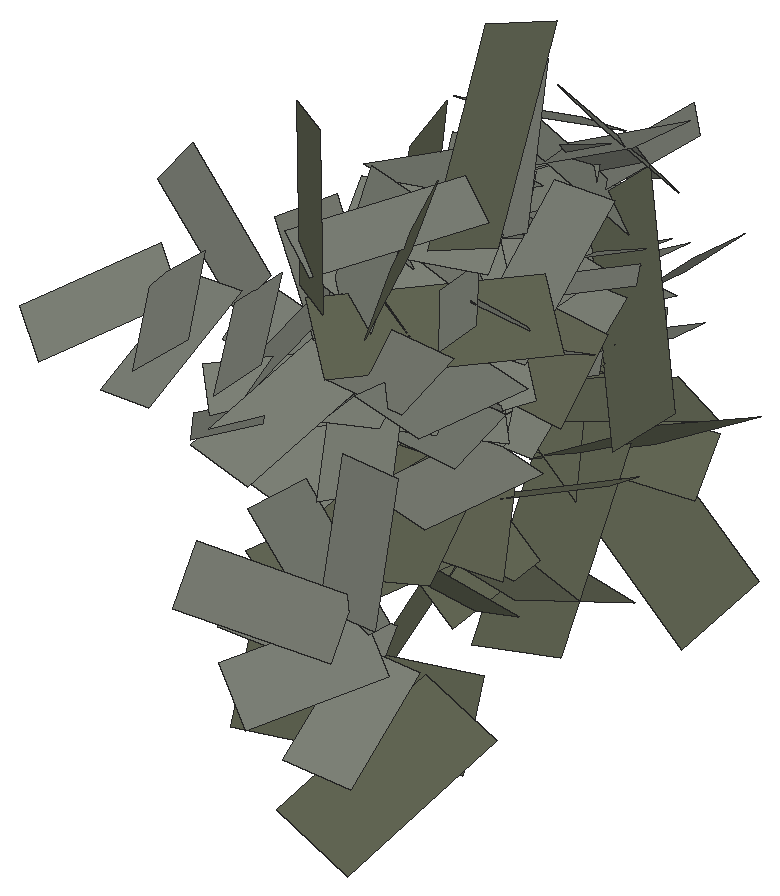
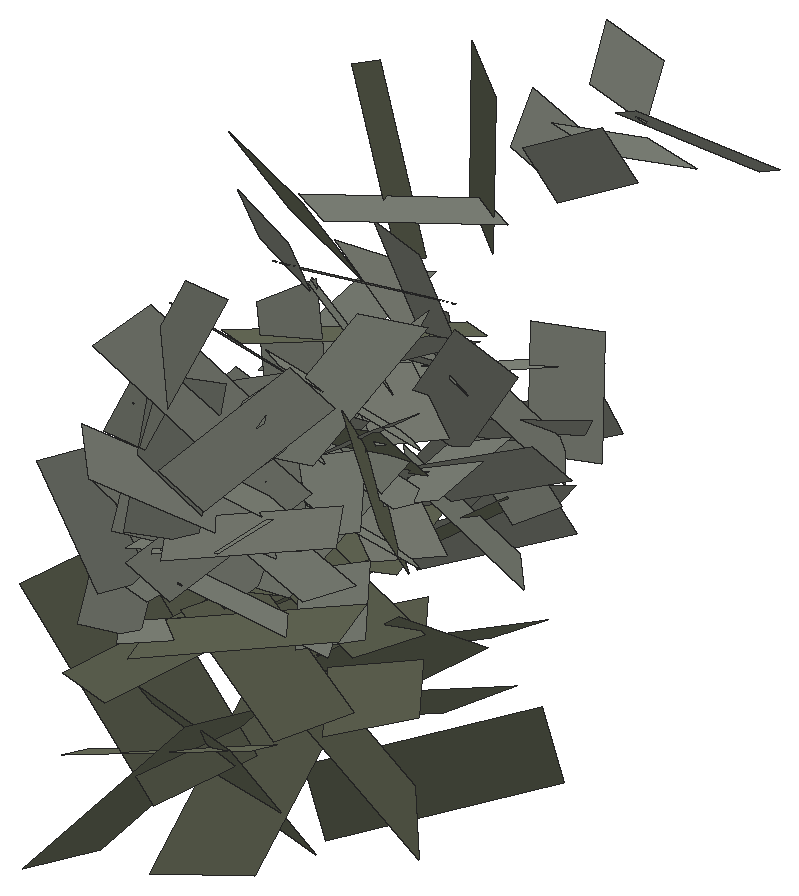
# SketchUp Ruby script. Lengths in inches.
U = 1.inch
M = Sketchup.active_model
def pt(a) = Geom::Point3d.new(a.map { |v| v * U })
def face(e, loops, mat)
  f = e.add_face(loops[0].map { |a| pt(a) })
  loops[1..].each { |l| e.add_face(l.map { |a| pt(a) }).erase! }
  f.material = f.back_material = mat if mat
  f
end
# faces: each face lists its corners as indices into pts; further lists are holes
def faces(e, pts, list, mat = nil) = list.each { |f| face(e, (f[0].is_a?(Array) ? f : [f]).map { |l| l.map { |i| pts[i] } }, mat) }
# xy, xz, yz: faces in a plane at the given z, y or x. An outline is a flat list of corners, or four numbers for a rectangle; further outlines are holes
def ring(l) = l.size == 4 ? [[l[0], l[1]], [l[2], l[1]], [l[2], l[3]], [l[0], l[3]]] : l.each_slice(2).to_a
def flat(e, list, mat, &to3) = list.each { |f| face(e, (f[0].is_a?(Array) ? f : [f]).map { |l| ring(l).map { |u, v| to3.(u, v) } }, mat) }
def xy(e, z, list, mat = nil) = flat(e, list, mat) { |x, y| [x, y, z] }
def xz(e, y, list, mat = nil) = flat(e, list, mat) { |x, z| [x, y, z] }
def yz(e, x, list, mat = nil) = flat(e, list, mat) { |y, z| [x, y, z] }
def lines(e, pts, list) = list.each { |a, b| e.add_line(pt(pts[a]), pt(pts[b])) }
# prism: a flat outline (further loops are holes) pulled along v
def prism(e, loops, v, mat = nil)
  f = face(e, loops, mat); d = Geom::Vector3d.new(v.map { |x| x * U })
  f.pushpull(f.normal.samedirection?(d) ? d.length : -d.length)
end
def box(e, o, s, mat = nil) = prism(e, [[o, [o[0] + s[0], o[1], o[2]], [o[0] + s[0], o[1] + s[1], o[2]], [o[0], o[1] + s[1], o[2]]]], [0, 0, s[2]], mat)
def at(x, y, z, deg = 0) = Geom::Transformation.translation(pt([x, y, z])) * Geom::Transformation.rotation(ORIGIN, Z_AXIS, deg.degrees)
def axes(o, x, y, z) = Geom::Transformation.new([*x, 0, *y, 0, *z, 0, *pt(o).to_a, 1])
def part(name) = M.definitions.add(name)
# library, detail: a bought-in or finely detailed component or shape, given as its bounding box
def library(name, o, s) = part(name).tap { |d| box(d.entities, o, s) }
def detail(e, o, s) = box(e.add_group.entities, o, s)
def put(e, d, t, mat = nil) = e.add_instance(d, t).tap { |i| i.material = mat if mat }
def group(e, t, mat = nil) = e.add_group.tap { |g| g.transformation = t; g.material = mat if mat }.entities
root = M.entities
M.materials.add("viburnumblaasdfas0df1w06d").color = [98, 102, 84]
M.materials.add("viburnumbladsadfasdfad0w122").color = [125, 129, 119]
c1 = part("Component\#315")
p = [[0.25,0,0],[2.05,0.01,0.35],[1.81,4.2,1.66],[0,4.19,1.3125]]
faces(c1.entities,p,[[0,1,2,3]],"viburnumbladsadfasdfad0w122")
c2 = part("viburnumblad2")
put(c2.entities,c1,axes([-19.23,-4.49,-32.18],[83.35428,0,0],[0,79.38502,0],[0,0,83.35428]))
c3 = part("Component\#314")
p = [[0.14,0,0],[2.58,0.05,0.25],[2.44,5.11,2.64],[0,5.05,2.39]]
faces(c3.entities,p,[[0,1,2,3]],"viburnumblaasdfas0df1w06d")
c4 = part("viburnumblad1\#2")
put(c4.entities,c3,axes([-37.25,6.23,19.31],[75.98784,0,0],[0,65.50676,0],[0,0,75.98784]))
put(root,c2,axes([2206.21,336.26,21.66],[0.00219,0.00955,0.00743],[-0.01307,0.00092,0.00265],[0.0015,-0.00837,0.01031]))
put(root,c4,axes([2205.43,338.76,20.89],[0.01183,-0.00442,0.01203],[-0.00182,0.01827,0.0085],[-0.01272,-0.00605,0.01028]))
put(root,c2,axes([2206.37,328.02,29.41],[-0.00814,0.00715,0.0046],[-0.00805,-0.00423,-0.00746],[-0.00268,-0.00803,0.00677]))
put(root,c2,axes([2204.18,344.4,21.67],[-0.01,-0.00652,-0.00001],[0.00542,-0.00831,-0.00274],[0.00166,-0.00256,0.01102]))
put(root,c2,axes([2202.71,334.87,22.83],[0.00888,-0.0091,-0.0009],[0.00823,0.00741,0.00631],[-0.00398,-0.00497,0.01104]))
put(root,c2,axes([2205.18,339.76,23.52],[-0.01211,-0.00173,0.00211],[0.00069,-0.01077,-0.00395],[0.00303,-0.00413,0.011]))
put(root,c2,axes([2206.93,346.05,25.19],[-0.0062,0.01038,-0.0034],[-0.01088,-0.00717,-0.00204],[-0.00346,0.00185,0.01194]))
put(root,c2,axes([2205.36,335.66,23.13],[0.01106,0.0052,0.00541],[-0.00756,0.007,0.00872],[0.00055,-0.01018,0.00865]))
put(root,c2,axes([2204.26,334.51,23.09],[-0.00865,-0.00796,-0.00491],[0.00846,-0.00952,0.00054],[-0.00401,-0.0029,0.01175]))
put(root,c2,axes([2202.83,344.76,22.0625],[0.00554,-0.00849,-0.00419],[0.01058,0.00621,0.0014],[0.00119,-0.0044,0.01049]))
put(root,c2,axes([2203.29,335.87,20],[0.00852,-0.00783,-0.00192],[0.00823,0.00741,0.00631],[-0.003,-0.00593,0.01088]))
put(root,c4,axes([2208.25,345.48,20.74],[-0.00473,0.01294,-0.00003],[-0.01473,-0.00539,-0.00308],[-0.0025,-0.00088,0.01352]))
put(root,c2,axes([2207.21,335.39,22.89],[-0.00749,0.00812,0.00752],[-0.01012,-0.00577,-0.00385],[0.00099,-0.00855,0.01022]))
put(root,c2,axes([2206.23,330.56,27.9],[0.00736,0.00309,0.0079],[-0.00921,0.00654,0.0057],[-0.00262,-0.00929,0.00521]))
put(root,c4,axes([2203.95,342.96,17.85],[-0.0111,-0.00766,0.00199],[0.00742,-0.01279,-0.00569],[0.00489,-0.00308,0.01206]))
put(root,c2,axes([2203.05,340.66,22.82],[0.00848,-0.00639,-0.00524],[0.0093,0.00903,0.00402],[0.00207,-0.0066,0.01002]))
put(root,c2,axes([2204.8125,343.71,24.35],[-0.00958,-0.00624,-0.00001],[0.00602,-0.00923,-0.00305],[0.00166,-0.00256,0.01102]))
put(root,c2,axes([2206.84,346.58,26.86],[-0.01136,0.00239,-0.0048],[-0.00314,-0.01208,0.00143],[-0.00434,0.00249,0.01152]))
put(root,c2,axes([2204.6,340.74,22.52],[-0.00866,-0.0095,-0.00259],[0.00823,-0.00655,-0.00374],[0.002,-0.00468,0.01099]))
put(root,c2,axes([2206.52,343.58,26.43],[-0.01523,0.00004,-0.00037],[-0.00005,-0.01523,0.00032],[-0.00037,0.00032,0.01523]))
put(root,c4,axes([2203.32,345.78,19.23],[-0.00529,-0.01137,-0.00003],[0.01295,-0.00601,-0.0028],[0.00218,-0.00104,0.01231]))
put(root,c2,axes([2203.52,344.16,24.8],[0.00577,-0.00885,-0.00437],[0.0098,0.00575,0.0013],[0.00119,-0.0044,0.01049]))
put(root,c2,axes([2203.8,344.5625,23.28],[-0.00269,-0.01067,-0.0031],[0.01162,-0.00239,-0.00186],[0.00104,-0.00341,0.01086]))
put(root,c4,axes([2207.89,338.85,15.1],[0.00636,0.01278,0.00656],[-0.01653,0.00548,0.00535],[0.00178,-0.00782,0.01351]))
put(root,c2,axes([2203.82,335.67,21.62],[0.00016,-0.01206,-0.00411],[0.01207,-0.0013,0.00429],[-0.00443,-0.00391,0.01129]))
put(root,c2,axes([2206.74,344.03,22.81],[-0.01389,0,-0.00185],[-0.00005,-0.01523,0.00032],[-0.00201,0.00032,0.0151]))
put(root,c2,axes([2203.82,339.62,25.59],[0.00883,-0.00666,-0.00546],[0.00861,0.00836,0.00373],[0.00207,-0.0066,0.01002]))
put(root,c2,axes([2207.31,338.52,23.91],[0.00207,0.01081,-0.00198],[-0.01024,0.00263,0.00364],[0.00398,0.00114,0.01039]))
put(root,c4,axes([2207.83,340.17,17.43],[-0.01218,0.00376,0.00725],[-0.00872,-0.0119,-0.00846],[0.0032,-0.00977,0.01045]))
put(root,c4,axes([2208.4,338.34,11.49],[-0.00011,0.00616,0.01357],[-0.0165,-0.00475,0.00202],[0.00445,-0.01294,0.00591]))
put(root,c4,axes([2204.5625,338.98,12.5],[0.01021,-0.01095,0.0021],[0.01009,0.01114,0.00903],[-0.00698,-0.00405,0.01279]))
put(root,c4,axes([2203.39,342.49,20.18],[-0.00229,-0.01326,-0.00295],[0.0155,-0.0021,-0.00237],[0.00206,-0.00324,0.01267]))
put(root,c2,axes([2207.49,336.78,22.07],[-0.0137,0.00216,0.00156],[-0.00229,-0.00943,-0.00711],[-0.00005,-0.00804,0.01068]))
put(root,c2,axes([2204.07,340.45,24.15],[0.00038,-0.01114,-0.00561],[0.01301,0.00109,-0.00087],[0.0016,-0.0057,0.01058]))
put(root,c2,axes([2208.21,344.95,23.86],[-0.00604,0.00926,-0.00001],[-0.00892,-0.00582,-0.00295],[-0.00247,-0.0016,0.01066]))
put(root,c2,axes([2206.62,338.78,22.62],[0.00864,0.00566,-0.00294],[-0.00615,0.01026,0.00169],[0.00342,0.0003,0.01064]))
put(root,c2,axes([2207.61,334.61,24.57],[-0.01312,0.00207,0.00149],[-0.00255,-0.01047,-0.0079],[-0.00005,-0.00804,0.01068]))
put(root,c2,axes([2205.34,339.6,25.21],[-0.00829,-0.0091,-0.00248],[0.00914,-0.00728,-0.00415],[0.002,-0.00468,0.01099]))
put(root,c2,axes([2207.84,346.66,23.85],[-0.01091,0.00229,-0.00461],[-0.00339,-0.01305,0.00154],[-0.00434,0.00249,0.01152]))
put(root,c2,axes([2207.37,329.4375,29.38],[-0.01118,0.00278,-0.00257],[-0.00011,-0.00839,-0.00838],[-0.00365,-0.00753,0.00688]))
put(root,c2,axes([2208.25,338.7,25.13],[-0.00607,0.00939,0.00026],[-0.0086,-0.00567,0.00435],[0.00378,0.00216,0.0103]))
put(root,c2,axes([2208.47,343.9,23.85],[0.00229,0.01091,-0.00461],[-0.01305,0.00339,0.00154],[0.00249,0.00434,0.01152]))
put(root,c2,axes([2205.38,335.26,25.11],[0.01312,-0.00207,-0.00149],[0.00246,0.00822,0.01025],[-0.00067,-0.01033,0.00845]))
put(root,c2,axes([2206.97,339.24,25.38],[0.009,0.00589,-0.00306],[-0.00569,0.0095,0.00156],[0.00342,0.0003,0.01064]))
put(root,c2,axes([2204.4375,344.84,24.53],[0.01077,-0.01075,-0.00083],[0.01118,0.01095,0.00335],[-0.00168,-0.00283,0.01488]))
put(root,c4,axes([2209.54,338.44,17.48],[-0.00702,0.01204,0.00725],[-0.01547,-0.00958,0.00093],[0.00442,-0.0058,0.01392]))
put(root,c2,axes([2206.23,344.98,24.57],[-0.01077,-0.01069,-0.00135],[0.00977,-0.00996,0.00094],[-0.00168,-0.00022,0.01514]))
put(root,c4,axes([2206.81,333.43,27.22],[0.01089,-0.00679,0.00142],[0.00218,0.00667,0.0129],[-0.00665,-0.00902,0.00468]))
put(root,c2,axes([2208.88,345.56,21.27],[-0.0063,0.00967,-0.00001],[-0.00803,-0.00524,-0.00265],[-0.00247,-0.0016,0.01066]))
put(root,c2,axes([2206.57,328.875,30.59],[-0.00766,-0.00322,-0.00823],[0.00764,-0.00813,-0.00386],[-0.0046,-0.00755,0.00633]))
put(root,c2,axes([2209.0625,337.48,21.01],[0.00051,0.01437,0.00412],[-0.01266,-0.00025,0.00242],[0.00266,-0.00396,0.0135]))
put(root,c2,axes([2209.23,344.41,25.26],[-0.007,0.00987,-0.00339],[-0.01018,-0.00558,0.00479],[0.00226,0.00542,0.01111]))
put(root,c4,axes([2206.66,341.1,12.74],[0.01682,-0.00022,0.00237],[-0.00091,0.01794,0.00812],[-0.00224,-0.00704,0.0153]))
put(root,c2,axes([2209.5,336.32,24.33],[0.00048,0.01376,0.00394],[-0.01406,-0.00028,0.00269],[0.00266,-0.00396,0.0135]))
put(root,c4,axes([2210.08,346.02,16.68],[-0.00341,0.01096,0.00392],[-0.01337,-0.00302,-0.00319],[-0.00164,-0.0045,0.01114]))
put(root,c2,axes([2207.33,347.42,25.26],[-0.00987,-0.007,-0.00339],[0.00558,-0.01018,0.00479],[-0.00542,0.00226,0.01111]))
put(root,c2,axes([2209.72,336.9,27.65],[-0.00274,0.01284,0.00559],[-0.01166,-0.00082,-0.00384],[-0.00348,-0.00589,0.01184]))
put(root,c4,axes([2207.95,345.11,13.125],[-0.01776,-0.00139,0.00308],[0.00179,-0.02087,0.00087],[0.003,0.001,0.0178]))
put(root,c4,axes([2205.85,339.49,19.81],[0.01107,-0.00525,0.00049],[0.00612,0.01279,-0.0012],[0,0.00115,0.01221]))
put(root,c2,axes([2208.5625,339.09,23.52],[-0.01065,0.00247,0.00234],[-0.00174,-0.01065,0.00331],[0.00294,0.00276,0.01043]))
put(root,c2,axes([2209.58,332.38,16.85],[-0.00011,0.00779,0.00854],[-0.01208,-0.00262,0.00224],[0.00345,-0.0089,0.00816]))
put(root,c2,axes([2205.41,345.15,26.5625],[0,-0.01516,-0.00154],[0.01507,-0.00022,0.00221],[-0.00223,-0.00152,0.015]))
put(root,c2,axes([2205.73,345.33,22.8],[0,-0.01583,-0.00161],[0.01357,-0.0002,0.00199],[-0.00223,-0.00152,0.015]))
put(root,c2,axes([2209.04,345.93,22.82],[-0.01032,0.0026,-0.00299],[-0.00231,-0.01123,-0.0018],[-0.0033,-0.001,0.0105]))
put(root,c2,axes([2207.39,336.5,23.99],[-0.01106,-0.0052,-0.00541],[0.00776,-0.00965,-0.0066],[-0.00127,-0.0082,0.01048]))
put(root,c2,axes([2206.71,339.63,23.89],[0.01065,-0.00247,-0.00234],[0.00251,0.01145,-0.00069],[0.00243,0.00013,0.01091]))
put(root,c2,axes([2210.1,336.46,29.55],[-0.01065,0.00857,-0.00023],[-0.00787,-0.00997,-0.00669],[-0.00415,-0.00484,0.01209]))
put(root,c4,axes([2211.27,339.14,22.42],[0.00121,0.01104,0.01007],[-0.01675,0.00403,-0.00241],[-0.00386,-0.00953,0.01091]))
put(root,c2,axes([2208.67,337.18,22.69],[0.01044,0.00958,0.00206],[-0.00879,0.00856,0.00474],[0.00211,-0.00514,0.0132]))
put(root,c2,axes([2210.35,337.27,22.625],[-0.00976,0.00988,0.00351],[-0.01076,-0.01049,-0.00039],[0.00219,-0.00277,0.01388]))
put(root,c2,axes([2207.46,330.97,29.29],[-0.00655,-0.0022,-0.00816],[0.00764,-0.00813,-0.00386],[-0.0054,-0.00785,0.00541]))
put(root,c4,axes([2207.74,339.58,20.09],[-0.01365,-0.00518,-0.0014],[0.0059,-0.01311,-0.00908],[0.00168,-0.00777,0.01232]))
put(root,c2,axes([2205.93,336.81,24.27],[0.00749,-0.00812,-0.00752],[0.01093,0.00403,0.00654],[-0.00171,-0.00982,0.0089]))
put(root,c2,axes([2209.99,330.04,18.7],[0.00026,0.00745,0.01011],[-0.01208,-0.00262,0.00224],[0.00344,-0.00977,0.00711]))
put(root,c2,axes([2208.97,331.39,18.08],[0.00896,0.00627,0.00619],[-0.00837,0.00305,0.00903],[0.00298,-0.01046,0.00629]))
put(root,c4,axes([2210.63,344.85,12.74],[0.00022,0.01682,0.00237],[-0.01794,-0.00091,0.00812],[0.00704,-0.00224,0.0153]))
put(root,c4,axes([2210.22,346.4,18.9],[-0.011,0.00511,-0.00003],[-0.00581,-0.01252,-0.00271],[-0.00101,-0.0021,0.0119]))
put(root,c4,axes([2206.93,339.24,15.14],[-0.00936,-0.00715,0.0061],[0.00985,-0.01174,0.00135],[0.00403,0.00472,0.01172]))
put(root,c4,axes([2211.625,338.39,25.09],[-0.01024,0.01003,0.00441],[-0.01249,-0.0094,-0.00763],[-0.00202,-0.00765,0.01274]))
put(root,c2,axes([2208.13,339.74,22.23],[-0.00842,-0.00565,0.00174],[0.00635,-0.00914,0.00106],[0.00096,0.00194,0.01097]))
put(root,c4,axes([2208.52,336.83,27.32],[0.01421,-0.00084,0.00442],[-0.0012,0.01582,0.00687],[-0.00438,-0.00595,0.01294]))
put(root,c2,axes([2209.83,345.45,26.51],[-0.01229,0.00259,0.00001],[-0.00225,-0.0107,0.00618],[0.00128,0.00604,0.01094]))
put(root,c2,axes([2206.66,337.9,23.05],[-0.00242,-0.00904,-0.00878],[0.01402,-0.00344,-0.00033],[-0.00196,-0.00893,0.00974]))
put(root,c2,axes([2208.64,337.89,27.8125],[0.01184,0.00091,0.00415],[-0.00322,0.01148,0.00668],[-0.0033,-0.00735,0.01104]))
put(root,c2,axes([2206.92,335.73,25.62],[-0.00252,-0.00942,-0.00914],[0.01298,-0.00318,-0.00031],[-0.00196,-0.00893,0.00974]))
put(root,c2,axes([2207,340.13,22.375],[0.00633,-0.0098,-0.00027],[0.00833,0.00542,-0.00155],[0.00159,0.00072,0.01104]))
put(root,c2,axes([2208.66,346.2,24.29],[-0.00856,-0.00558,-0.00422],[0.00556,-0.00947,0.00126],[-0.00425,-0.00115,0.01014]))
put(root,c4,axes([2206.18,340.06,17.63],[0.00308,-0.0114,0.00333],[0.01375,0.00318,-0.00182],[0.00071,0.00361,0.0117]))
put(root,c2,axes([2210.72,331.62,17.86],[-0.00859,0.00427,0.00811],[-0.00794,-0.00683,-0.00482],[0.00302,-0.00917,0.00803]))
put(root,c4,axes([2210.09,336.98,13.64],[-0.01186,-0.00066,0.00699],[-0.00532,-0.01121,-0.01007],[0.00532,-0.0098,0.0081]))
put(root,c2,axes([2208.16,338.63,21.51],[0.01298,0.00037,-0.00224],[0.00059,0.01317,0.00559],[0.0024,-0.0056,0.01296]))
put(root,c2,axes([2207.7,340.41,23.52],[-0.00207,-0.01081,0.00198],[0.01001,-0.00209,-0.00093],[0.00139,0.00174,0.01096]))
put(root,c2,axes([2208.73,339.99,24.83],[-0.009,-0.00589,0.00306],[0.00635,-0.00914,0.00106],[0.00195,0.00259,0.0107]))
put(root,c4,axes([2206.71,346.35,16.39],[-0.00613,-0.01546,0.00166],[0.01796,-0.00686,0.00247],[-0.00138,0.00232,0.01649]))
put(root,c2,axes([2207.45,340.53,25.08],[0.00607,-0.00939,-0.00026],[0.00926,0.00603,-0.00173],[0.00159,0.00072,0.01104]))
put(root,c2,axes([2209.23,346.87,21.65],[-0.00821,-0.00536,-0.00406],[0.00601,-0.01023,0.00136],[-0.00425,-0.00115,0.01014]))
put(root,c2,axes([2210.49,338.6,21.19],[-0.01371,0.0002,0.00098],[-0.0004,-0.01527,-0.00242],[0.00098,-0.00226,0.01411]))
put(root,c2,axes([2208.51,337.75,24.8125],[0.01428,-0.00021,-0.00102],[0.00059,0.01317,0.00559],[0.00086,-0.00561,0.01315]))
put(root,c4,axes([2208.0625,335.4,27.16],[0.00428,-0.01029,-0.00658],[0.01194,-0.00078,0.00879],[-0.00649,-0.00737,0.00685]))
put(root,c2,axes([2208.4375,347.03,22.88],[-0.00178,-0.0105,-0.00298],[0.00981,-0.00286,0.00422],[-0.00478,-0.00196,0.00978]))
put(root,c2,axes([2210.64,333.07,17.35],[-0.01296,-0.00148,0.00142],[-0.00002,-0.00776,-0.00823],[0.00196,-0.00903,0.00851]))
put(root,c4,axes([2211.09,341.61,20.21],[0.01304,-0.00033,0.00964],[-0.00605,0.01553,0.00873],[-0.00811,-0.00915,0.01066]))
put(root,c2,axes([2211.01,337.3,24.51],[-0.01428,0.00021,0.00102],[-0.00037,-0.01414,-0.00224],[0.00098,-0.00226,0.01411]))
put(root,c2,axes([2209.11,330.7,19.84],[0.01241,0.00141,-0.00136],[0.00049,0.00618,0.01093],[0.0019,-0.01085,0.00605]))
